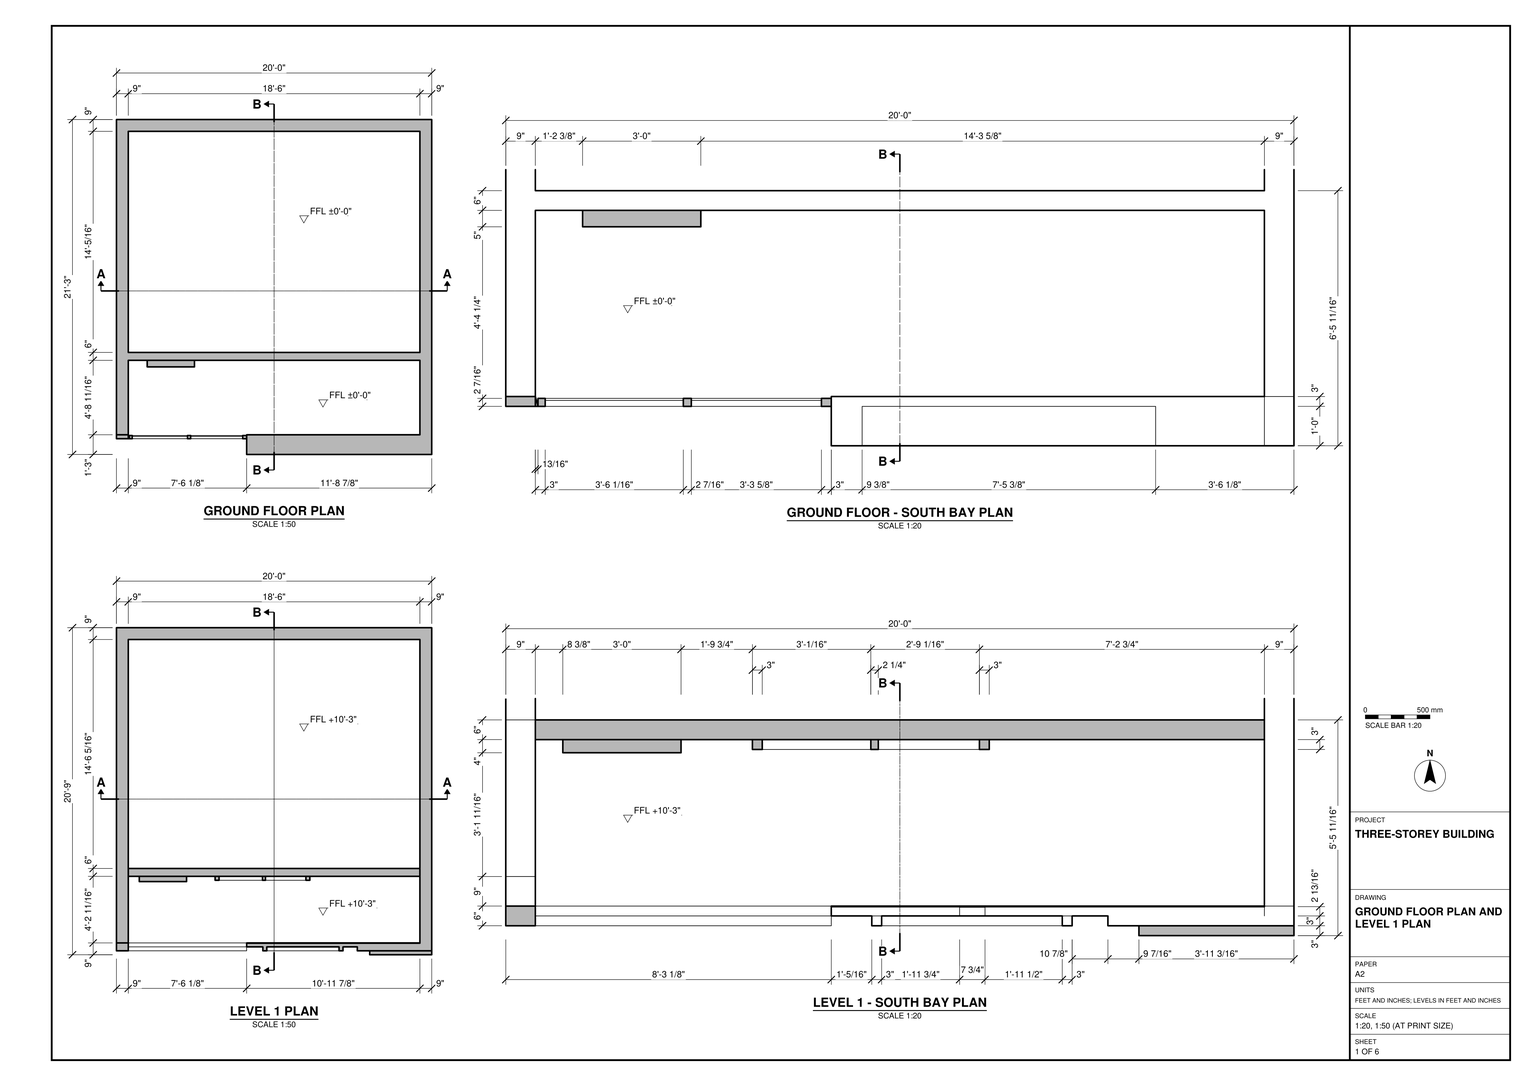
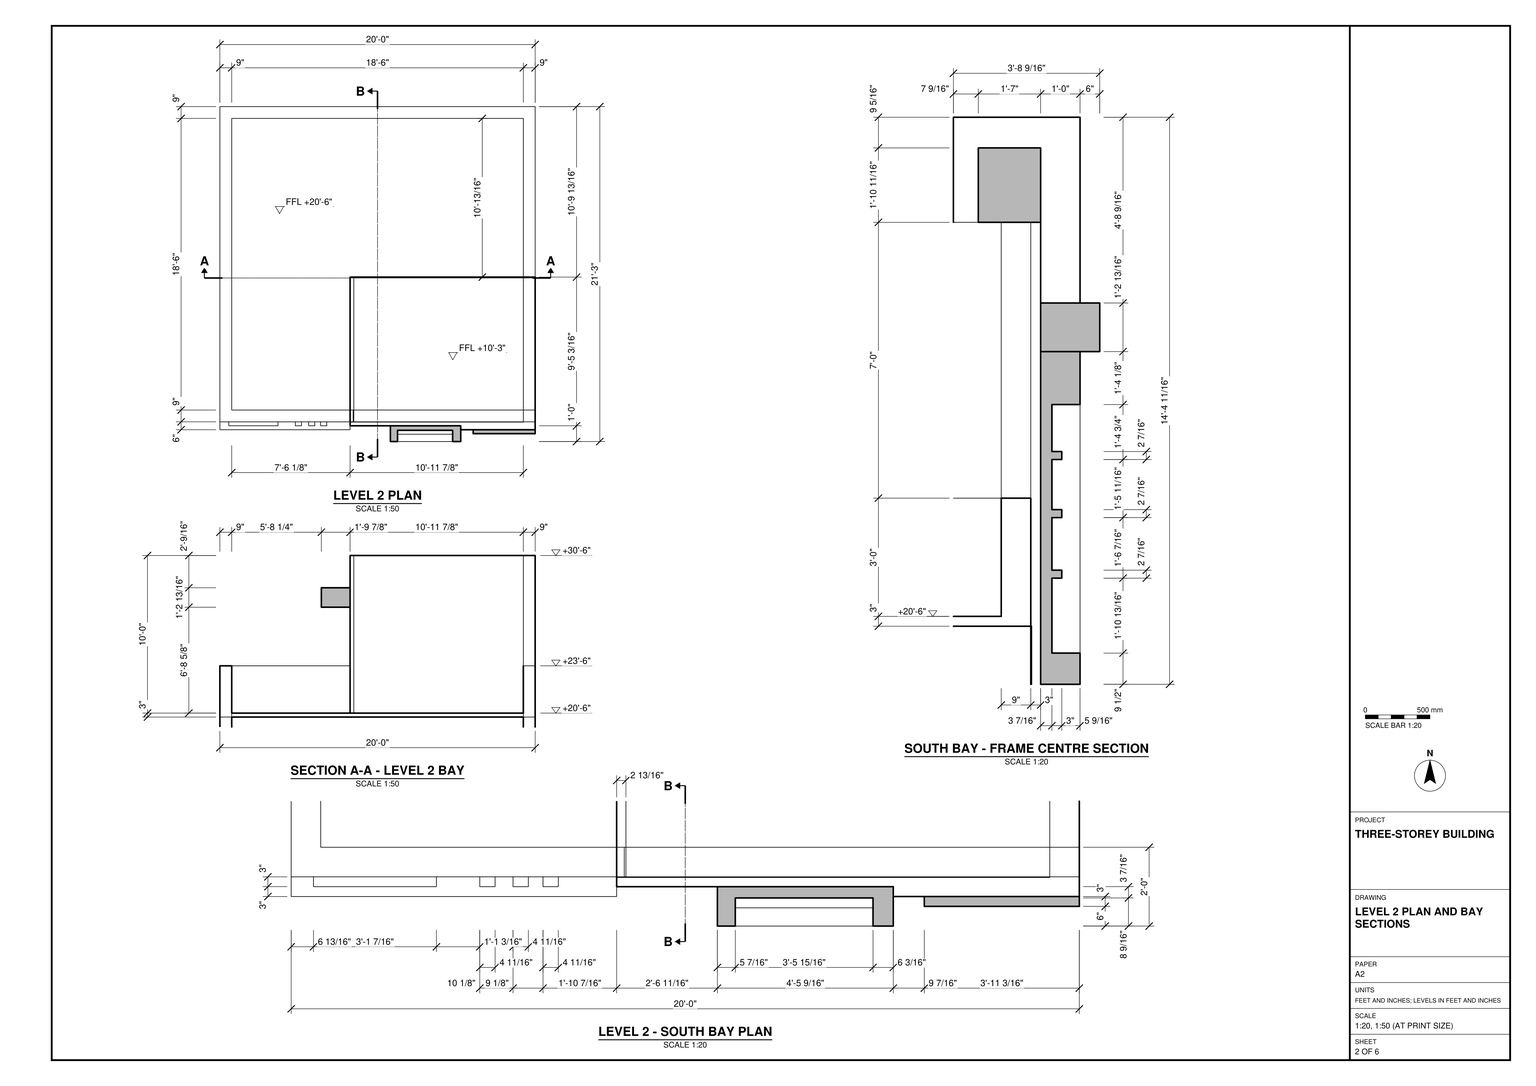
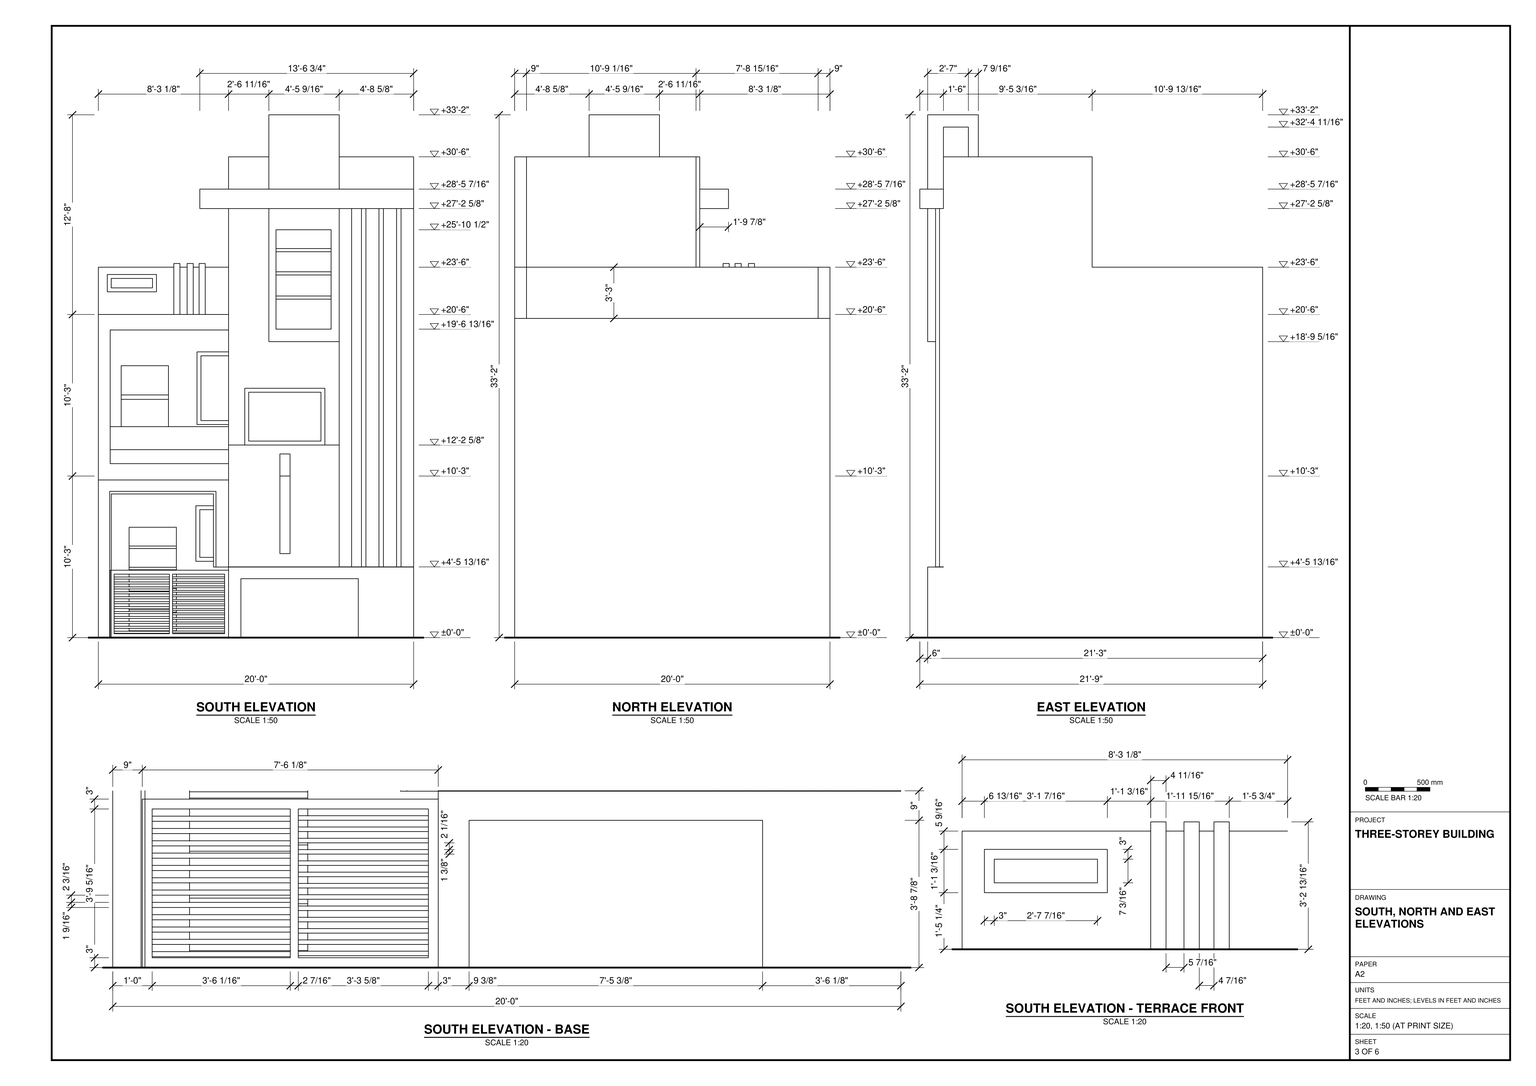
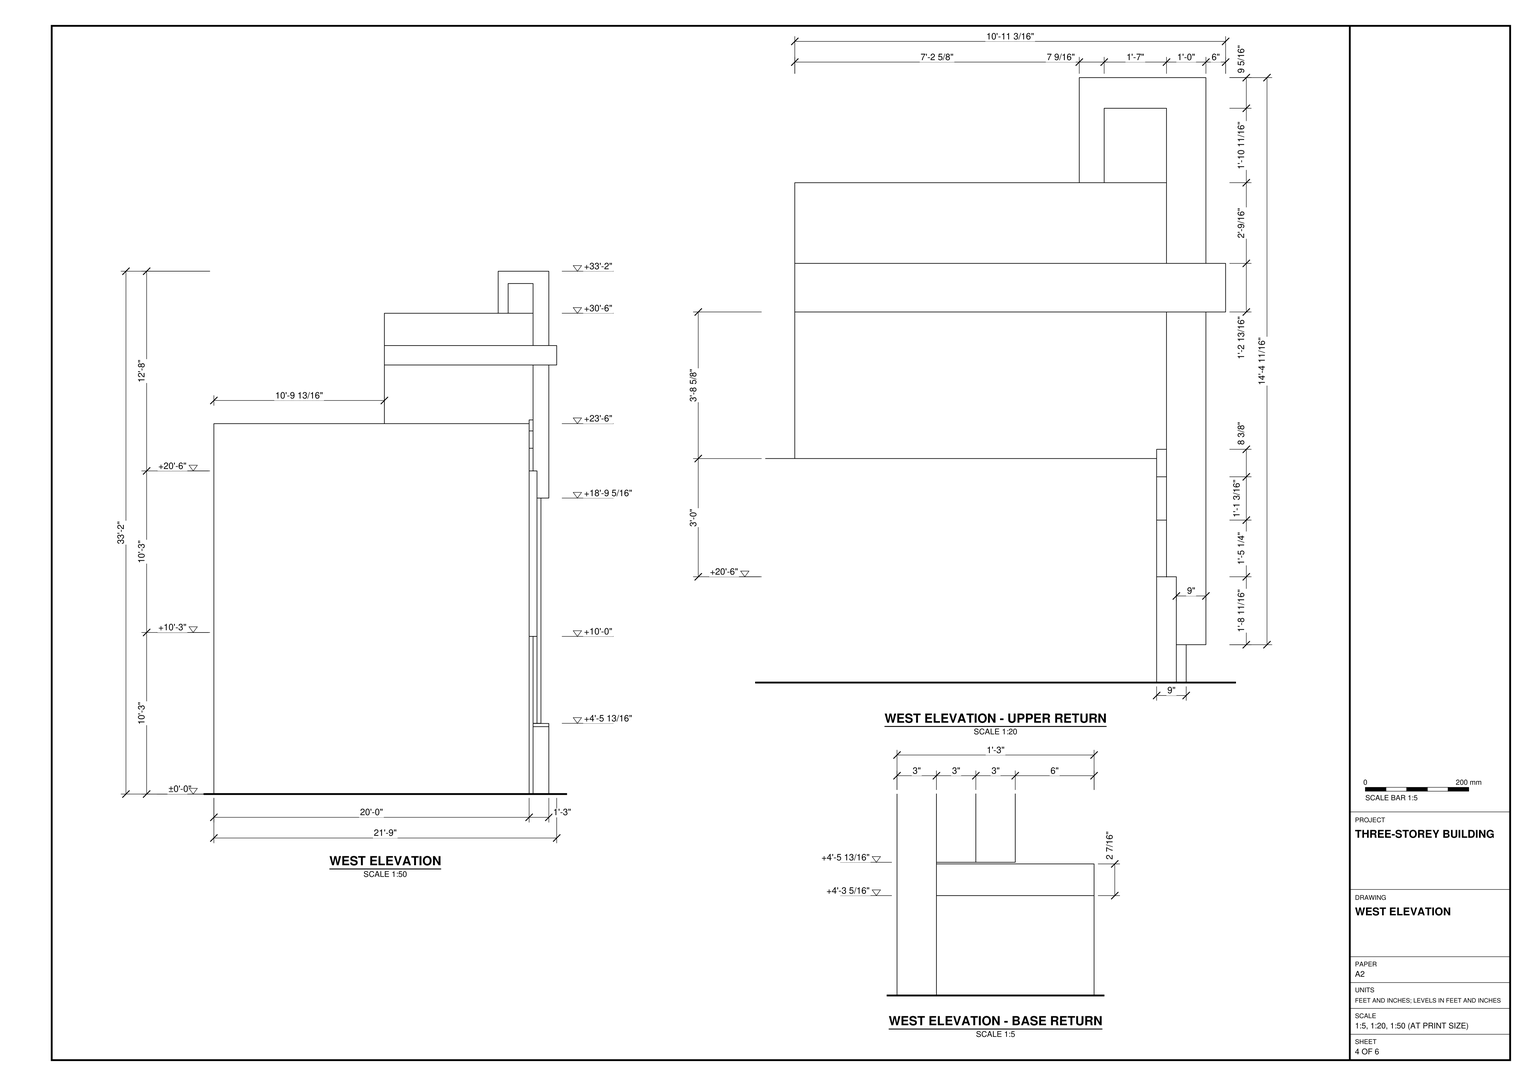
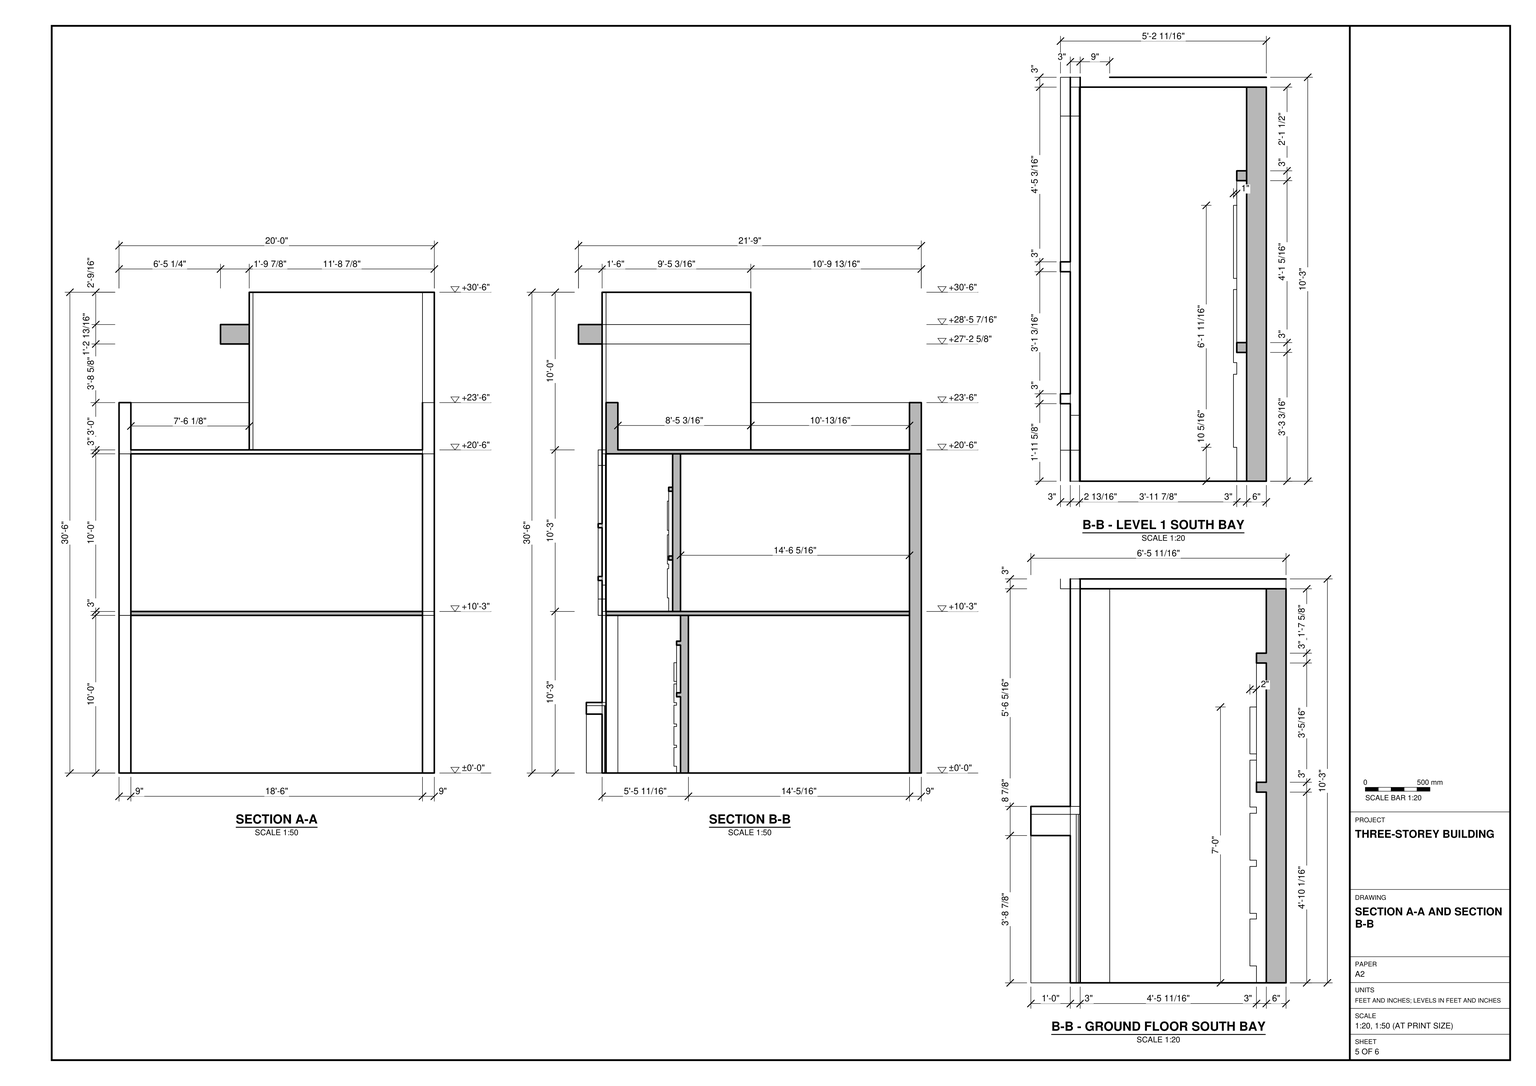
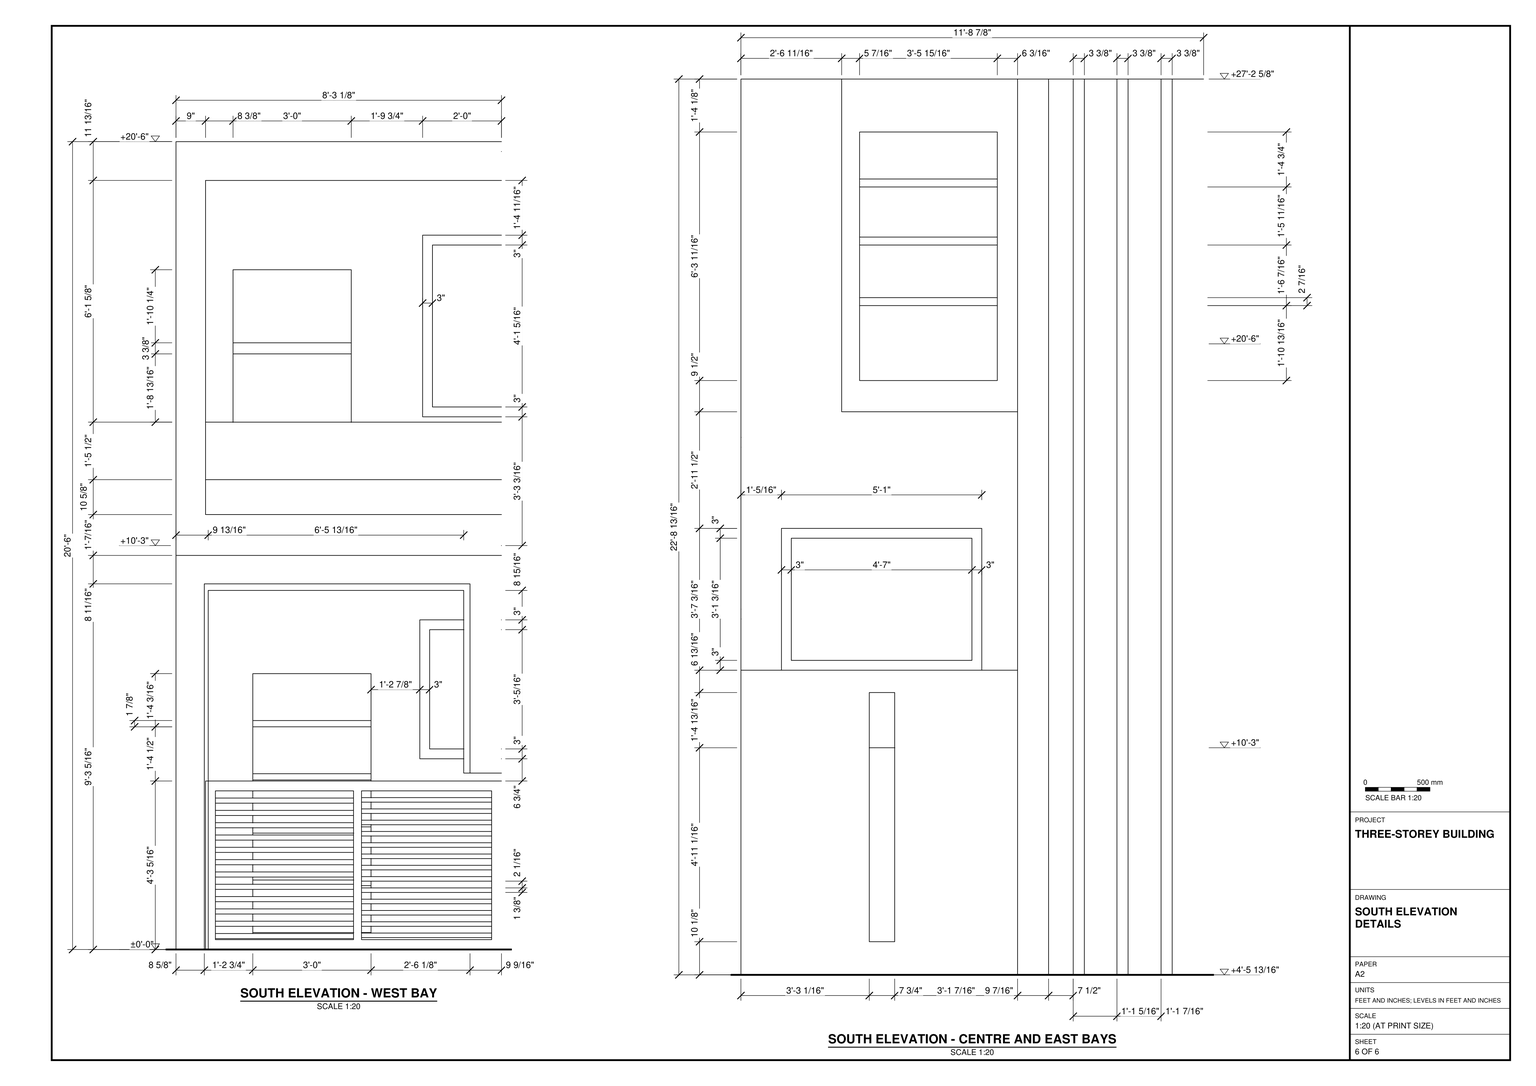
Build the three-storey building in SketchUp from task_files/diagram_01.pdf. Work in feet and inches. Set the overall width to 20'-0", the depth including the south façade projections to 21'-9", and the height to 33'-2". Set the ground floor at ±0'-0", Level 1 at +10'-3", and Level 2 at +20'-6".

Use the floor plans to lay out the main enclosure and the shallow bay along its south side. Model the 9" perimeter walls and the 6" transverse walls where dimensioned. Follow the sections for the floor slabs, flat roof, terrace parapet and taller volume at the southeast corner. Use the enlarged bay plans with the south elevation to place the openings, frames and projections at their correct depths. On the left, model the slatted gate and the recessed bays behind and above it. On the right, include the solid base, tall vertical fins, raised rectangular frame and projecting horizontal band. Carry the terrace-front details around only as far as the plans show.

Keep walls, slabs and roof elements in separate groups or components, and do the same for each furniture or joinery piece shown. Use components for repeated parts. Decor and loose items may be any suitable library components. Save one SketchUp model as output_files/three_storey_building_with_a_recessed_south_bay.skp.

# SketchUp Ruby script. Lengths in inches.
U = 1.inch
M = Sketchup.active_model
def pt(a) = Geom::Point3d.new(a.map { |v| v * U })
def face(e, loops, mat)
  f = e.add_face(loops[0].map { |a| pt(a) })
  loops[1..].each { |l| e.add_face(l.map { |a| pt(a) }).erase! }
  f.material = f.back_material = mat if mat
  f
end
# faces: each face lists its corners as indices into pts; further lists are holes
def faces(e, pts, list, mat = nil) = list.each { |f| face(e, (f[0].is_a?(Array) ? f : [f]).map { |l| l.map { |i| pts[i] } }, mat) }
# xy, xz, yz: faces in a plane at the given z, y or x. An outline is a flat list of corners, or four numbers for a rectangle; further outlines are holes
def ring(l) = l.size == 4 ? [[l[0], l[1]], [l[2], l[1]], [l[2], l[3]], [l[0], l[3]]] : l.each_slice(2).to_a
def flat(e, list, mat, &to3) = list.each { |f| face(e, (f[0].is_a?(Array) ? f : [f]).map { |l| ring(l).map { |u, v| to3.(u, v) } }, mat) }
def xy(e, z, list, mat = nil) = flat(e, list, mat) { |x, y| [x, y, z] }
def xz(e, y, list, mat = nil) = flat(e, list, mat) { |x, z| [x, y, z] }
def yz(e, x, list, mat = nil) = flat(e, list, mat) { |y, z| [x, y, z] }
def lines(e, pts, list) = list.each { |a, b| e.add_line(pt(pts[a]), pt(pts[b])) }
# prism: a flat outline (further loops are holes) pulled along v
def prism(e, loops, v, mat = nil)
  f = face(e, loops, mat); d = Geom::Vector3d.new(v.map { |x| x * U })
  f.pushpull(f.normal.samedirection?(d) ? d.length : -d.length)
end
def box(e, o, s, mat = nil) = prism(e, [[o, [o[0] + s[0], o[1], o[2]], [o[0] + s[0], o[1] + s[1], o[2]], [o[0], o[1] + s[1], o[2]]]], [0, 0, s[2]], mat)
def at(x, y, z, deg = 0) = Geom::Transformation.translation(pt([x, y, z])) * Geom::Transformation.rotation(ORIGIN, Z_AXIS, deg.degrees)
def axes(o, x, y, z) = Geom::Transformation.new([*x, 0, *y, 0, *z, 0, *pt(o).to_a, 1])
def part(name) = M.definitions.add(name)
# library, detail: a bought-in or finely detailed component or shape, given as its bounding box
def library(name, o, s) = part(name).tap { |d| box(d.entities, o, s) }
def detail(e, o, s) = box(e.add_group.entities, o, s)
def put(e, d, t, mat = nil) = e.add_instance(d, t).tap { |i| i.material = mat if mat }
def group(e, t, mat = nil) = e.add_group.tap { |g| g.transformation = t; g.material = mat if mat }.entities
root = M.entities
M.materials.add("[0004_HotPink]").color = [193, 79, 136]
M.materials.add("[0022_Maroon]").color = [128, 0, 0]
M.materials.add("[0079_Teal]").color = [0, 104, 104]
M.materials.add("[Color B07]").color = [153, 38, 0]
M.materials.add("[Color B08]").color = [63, 15, 0]
M.materials.add("[Color H08]").color = [0, 102, 102]
M.materials.add("[Color L03]").color = [206, 81, 144]
M.materials.add("[Color M05]").color = [114, 114, 114]
M.materials.add("[Color M09]").color = [0, 0, 0]
M.materials.add("[Formica Beige]").color = [211, 187, 149]
M.materials.add("[Formica Speckled Grey]").color = [94, 105, 111]
M.materials.add("[Translucent Glass Blue]").color = [67, 100, 160]
M.materials["[Translucent Glass Blue]"].alpha = 0.5
M.materials.add("[Translucent Glass Gray]").color = [198, 161, 76]
M.materials["[Translucent Glass Gray]"].alpha = 0.5
M.materials.add("[Wood Floor Parquet]").color = [122, 75, 32]
xy(root,0,[[99.11,6,99.11,21,231,21,231,6,197.89,6,197.89,18,108.51,18,108.51,6],[231,6,240,21],[0,18,9,21],[9,18,9,21,9.32,19.8125,9.32,18],[9.81,18,9.81,20.4375,99.11,20.4375,99.11,21,231,21,231,77.6875,59.39,77.6875,59.39,74.6875,23.39,74.6875,23.39,77.6875,9,77.6875,9,21,9.32,19.8125],
  [9.32,18,9.32,19.8125,9.81,18],[9.81,18,99.11,19.8125],[9.81,19.8125,99.11,20.4375],[[0,21,0,261,240,261,240,21,231,21,231,77.6875,9,77.6875,9,21],[9,83.6875,231,252]],[23.39,74.6875,59.39,77.6875],
  [9,83.6875,231,252]])
xy(root,3,[[12,19.8125,54.06,20.4375],[56.5,19.8125,96.11,20.4375]])
xy(root,3,[[12,18,54.06,19.8125],[56.5,18,96.11,19.8125]],"[Color M09]")
xy(root,5.15,[[23.39,72.6875,59.39,74.6875]])
xy(root,19.4375,[[23.39,72.6875,59.39,74.6875]],"[Color B08]")
xy(root,21.15,[[23.39,72.6875,59.39,74.6875]],"[Color B08]")
xy(root,34.86,[[12,19.8125,54.06,20.4375]])
xy(root,35.4375,[[23.39,72.6875,59.39,74.6875]],"[Color B08]")
xy(root,37.06,[[12,19.8125,54.06,20.4375]])
xy(root,37.34,[[23.39,72.6875,59.39,74.6875]],"[Color B08]")
xy(root,38.61,[[12,19.8125,54.06,20.4375]])
xy(root,40.81,[[12,19.8125,54.06,20.4375]])
xy(root,42.36,[[12,19.8125,54.06,20.4375]])
xy(root,44.56,[[12,19.8125,54.06,20.4375]])
xy(root,44.85,[[108.51,6,197.89,18]])
xy(root,46.11,[[12,19.8125,54.06,20.4375]])
xy(root,48.31,[[56.5,19.8125,96.11,20.4375]])
xy(root,48.31,[[12,18,54.06,20.4375],[56.5,18,96.11,19.8125]],"[Color M09]")
xy(root,51.31,[[9,18,9.81,18,9.81,20.4375,99.11,20.4375,99.11,21,9,21]])
xy(root,51.31,[[9.81,18,99.11,20.4375]],"[Color M09]")
xy(root,51.625,[[23.39,72.6875,59.39,74.6875]],"[Color B08]")
xy(root,53.53,[[23.39,72.6875,59.39,74.6875]],"[Color B08]")
xy(root,53.72,[[99.11,6,240,18],[87.61,18,99.11,21]])
xy(root,53.84,[[192.79,12,240,15],[183.35,15,240,18]])
xy(root,58.07,[[74.24,74.6875,126.74,77.6875]],"[Color B07]")
xy(root,61.07,[[77.24,74.6875,100.49,77.6875],[102.23,74.6875,123.74,77.6875]],"[Color B07]")
xy(root,63.9375,[[138.2,18,145.93,20.625]],"[Color L03]")
xy(root,67.8125,[[23.39,72.6875,59.39,74.6875]],"[Color B08]")
xy(root,69.72,[[23.39,72.6875,59.39,74.6875]],"[Color B08]")
xy(root,84,[[23.39,72.6875,59.39,77.6875]],"[Color B08]")
xy(root,97.39,[[77.24,74.6875,100.49,77.6875],[102.23,74.6875,123.74,77.6875]],"[Color B07]")
xy(root,100.39,[[74.24,74.6875,126.74,77.6875]],"[Color B07]")
xy(root,109.34,[[9.81,18,9,21,87.61,21,87.61,18]])
xy(root,120,[[0,15,9,18],[9,15,99.11,18],[0,18,99.11,21],[9,21,231,77.6875],[9,77.6875,231,83.6875],
  [9,83.6875,231,252]])
xy(root,123,[[99.11,20.8125,231,21],[9,21,231,21,231,71.6875,53.37,71.6875,53.37,68.6875,17.37,68.6875,17.37,71.6875,9,71.6875],[17.37,68.6875,53.37,71.6875],[9,71.6875,231,77.6875],[9,77.6875,231,252]])
xy(root,132.44,[[9,15,99.11,18],[9,18,99.11,21]])
xy(root,133.3125,[[17.37,67.6875,53.37,68.6875]])
xy(root,139.82,[[138.2,18,145.93,20.625]],"[Color L03]")
xy(root,143.07,[[9,18,99.11,21]])
xy(root,146.61,[[111.45,15,172.45,18]])
xy(root,149.61,[[114.45,15,169.45,18]])
xy(root,155.5625,[[17.37,67.6875,53.37,68.6875]],"[Color B08]")
xy(root,159.125,[[17.37,67.6875,53.37,68.6875]])
xy(root,162.21,[[75.1,68.6875,147.22,71.6875]])
xy(root,165.21,[[78.1,68.6875,111.16,71.6875],[113.44,68.6875,144.22,71.6875]],"[Color B07]")
xy(root,181.375,[[17.37,67.6875,53.37,68.6875]],"[Color B08]")
xy(root,184.75,[[17.37,67.6875,53.37,68.6875]],"[Color B08]")
xy(root,186.8,[[114.45,15,169.45,18]])
xy(root,189.8,[[111.45,15,172.45,18]])
xy(root,207,[[17.37,67.6875,53.37,71.6875]],"[Color B08]")
xy(root,214.52,[[78.1,68.6875,111.16,71.6875],[113.44,68.6875,144.22,71.6875]],"[Color B07]")
xy(root,217.52,[[75.1,68.6875,147.22,71.6875]],"[Color B07]")
xy(root,225.3125,[[129.79,6,183.35,18]],"[Color L03]")
xy(root,234.1875,[[9,15,99.11,21]])
xy(root,234.82,[[135.24,6,177.18,14.5625]],"[Color L03]")
xy(root,243,[[99.11,20.8125,231,21],[9,21,231,71.6875],[9,71.6875,231,77.6875],[9,77.6875,231,252],[9,252,231,252.125],
  [9,252.125,231,261]])
xy(root,246,[[0,15,99.11,15,99.11,21,81.35,21,81.35,18,76.69,18,76.69,21,72.22,21,72.22,18,67.56,18,67.56,21,62.1,21,62.1,18,57.44,18,57.44,21,0,21],[57.44,18,62.1,21],[67.56,18,72.22,21],[76.69,18,81.35,21],[9,30,99.11,30,99.11,131.1875,231,131.1875,231,252,9,252],
  [99.11,30,101.9375,131.1875],[101.9375,30,231,131.1875]])
xy(root,257.65,[[135.24,11.5625,177.18,14.5625]],"[0022_Maroon]")
xy(root,260.07,[[135.24,11.5625,177.18,14.5625]],"[0022_Maroon]")
xy(root,263.25,[[6.79,18,44.23,21]])
xy(root,266.25,[[9.79,18,41.23,30]])
xy(root,273.4375,[[9.79,18,41.23,30]])
xy(root,276.08,[[135.24,11.5625,177.18,14.5625]],"[0022_Maroon]")
xy(root,276.4375,[[6.79,18,44.23,21]])
xy(root,278.51,[[135.24,11.5625,177.18,14.5625]],"[0022_Maroon]")
xy(root,282,[[0,21,99.11,21,99.11,30,9,30,9,252,231,252,231,131.1875,240,131.1875,240,261,0,261],[99.11,21,101.4375,30],[101.4375,21,101.9375,30],[101.9375,21,231,30]])
xy(root,284.8125,[[57.44,18,62.1,21],[67.56,18,72.22,21],[76.69,18,81.35,21]],"[Formica Speckled Grey]")
xy(root,293.77,[[135.24,11.5625,177.18,14.5625]],"[0022_Maroon]")
xy(root,296.2,[[135.24,11.5625,177.18,14.5625]],"[0022_Maroon]")
xy(root,310.51,[[135.24,6,177.18,14.5625]],"[Color L03]")
xy(root,326.63,[[77.24,0,77.24,131.1875,99.11,131.1875,99.11,18,129.79,18,129.79,6,183.35,6,183.35,15,192.79,15,192.79,12,240,12,240,0],[129.79,6,183.35,18],[192.79,12,240,15],[183.35,15,240,18]])
xy(root,341.43,[[77.24,0,240,0,240,18,183.35,18,183.35,6,129.79,6,129.79,18,99.11,18,99.11,131.1875,77.24,131.1875],[129.79,6,183.35,18]])
xy(root,366,[[[99.11,18,240,131.1875],[129.79,36.98,183.35,44.5625]]],"[0079_Teal]")
xy(root,388.66,[[129.79,18,183.35,36.98]],"[0004_HotPink]")
xy(root,398,[[129.79,6,183.35,44.5625]],"[0004_HotPink]")
xz(root,0,[[77.24,326.63,240,341.43]])
xz(root,6,[[99.11,0,108.51,0,108.51,44.85,197.89,44.85,197.89,0,240,0,240,53.72,99.11,53.72]])
xz(root,6,[[[129.79,225.3125,183.35,326.63],[135.24,234.82,177.18,310.51]],[129.79,341.43,183.35,398]],"[Color L03]")
xz(root,11.5625,[[135.24,257.65,177.18,260.07],[135.24,276.08,177.18,278.51],[135.24,293.77,177.18,296.2]],"[0022_Maroon]")
xz(root,12,[[200.3,53.84,203.68,326.63],[213.61,53.84,216.99,326.63],[227.05,53.84,230.43,326.63]])
xz(root,12,[[192.79,53.84,200.3,326.63],[203.68,53.84,213.61,326.63],[216.99,53.84,227.05,326.63],[230.43,53.84,240,326.63]],"[Color M05]")
xz(root,14.5625,[[135.24,234.82,177.18,257.65],[135.24,260.07,177.18,276.08],[135.24,278.51,177.18,293.77],[135.24,296.2,177.18,310.51]],"[Translucent Glass Blue]")
xz(root,15,[[192.79,53.84,240,326.63],[0,120,99.11,120,99.11,132.44,9,132.44,9,234.1875,99.11,234.1875,99.11,246,0,246],[[111.45,146.61,172.45,189.8],[114.45,149.61,169.45,186.8]]])
xz(root,15,[[183.35,53.84,192.79,326.63]],"[Color M05]")
xz(root,18,[[8.62,0,9,0,9,51.31,9.81,51.31,9.81,109.34,87.61,109.34,87.61,53.72,89.53,53.72,89.53,111.34,8.62,111.34],[9,0,9.81,51.31],[99.11,53.72,108.51,53.84],[108.51,53.72,240,53.84],[114.45,149.61,169.45,186.8],
  [129.79,225.3125,183.35,326.63],[[6.79,263.25,44.23,276.4375],[9.79,266.25,41.23,273.4375]],[99.11,326.63,129.79,341.43],[129.79,326.63,183.35,341.43],[183.35,326.63,240,341.43],
  [129.79,341.43,183.35,366]])
xz(root,18,[[129.79,366,183.35,388.66]],"[0004_HotPink]")
xz(root,18,[[99.11,146.61,111.45,146.61,111.45,189.8,172.45,189.8,172.45,146.61,183.35,146.61,183.35,225.3125,129.79,225.3125,129.79,326.63,99.11,326.63],[99.11,341.43,129.79,366],[183.35,341.43,240,366]],"[0079_Teal]")
xz(root,18,[[0,0,8.62,0,8.62,111.34,89.53,111.34,89.53,53.72,99.11,53.72,99.11,120,0,120]],"[Color H08]")
xz(root,18,[[[99.11,53.84,183.35,146.61],[138.2,63.9375,145.93,139.82]]],"[Color L03]")
xz(root,18,[[[9.81,0,99.11,51.31],[12,3,54.06,48.31],[56.5,3,96.11,48.31]]],"[Color M09]")
xz(root,18,[[57.44,246,62.1,284.8125],[67.56,246,72.22,284.8125],[76.69,246,81.35,284.8125]],"[Formica Speckled Grey]")
xz(root,18,[[9,143.07,99.11,160.59]],"[Translucent Glass Blue]")
xz(root,18,[[108.51,0,197.89,44.85],[9,132.44,99.11,143.07]],"[Wood Floor Parquet]")
xz(root,19.8125,[[12,1.11,54.06,3],[56.5,1.5625,96.11,3],[12,3,54.06,3.31],[56.5,3,96.11,3.62],[12,3.31,54.06,4.86],
  [56.5,3.62,96.11,5],[12,7.06,54.06,8.61],[56.5,7.06,96.11,8.4375],[56.5,10.49,96.11,11.875],[12,10.81,54.06,12.36],
  [56.5,13.93,96.11,15.3125],[12,14.56,54.06,16.11],[56.5,17.37,96.11,18.75],[12,18.31,54.06,19.86],[56.5,20.81,96.11,22.1875],
  [12,22.06,54.06,23.61],[56.5,24.24,96.11,25.625],[12,25.81,54.06,27.36],[56.5,27.68,96.11,29.0625],[12,29.56,54.06,31.11],
  [56.5,31.12,96.11,32.5],[12,33.31,54.06,34.86],[56.5,34.56,96.11,35.9375],[12,37.06,54.06,38.61],[56.5,37.99,96.11,39.375],
  [12,40.81,54.06,42.36],[56.5,41.43,96.11,42.8125],[12,44.56,54.06,46.11],[56.5,44.87,96.11,46.25]])
xz(root,20.4375,[[[9.81,0,99.11,51.31],[12,3,54.06,48.31],[56.5,3,96.11,48.31]]])
xz(root,20.625,[[138.2,63.9375,145.93,139.82]])
xz(root,20.8125,[[99.11,123,231,243]])
xz(root,21,[[0,0,9,120],[99.11,0,231,120],[87.61,53.72,99.11,109.34],[0,120,9,242.93],[9,120,99.11,123],
  [99.11,120,231,123],[9,123,99.11,132.44],[99.11,123,231,243],[9,132.44,99.11,143.07],[9,234.1875,99.11,242.93],
  [0,242.93,0,246,99.11,246,99.11,243,9,243,9,242.93],[9,242.93,99.11,243],[99.11,243,231,282],[57.44,246,62.1,282],[67.56,246,72.22,282],
  [76.69,246,81.35,282],[57.44,282,62.1,284.8125],[67.56,282,72.22,284.8125],[76.69,282,81.35,284.8125]])
xz(root,21,[[[0,246,57.44,282],[6.79,263.25,44.23,276.4375]],[62.1,246,67.56,282],[72.22,246,76.69,282],[81.35,246,99.11,282]],"[Formica Beige]")
xz(root,30,[[[9,246,99.11,282],[9.79,266.25,41.23,273.4375]],[99.11,246,101.9375,282],[101.9375,246,231,282]])
xz(root,36.98,[[129.79,366,183.35,388.66]],"[0004_HotPink]")
xz(root,44.5625,[[129.79,366,183.35,398]])
xz(root,67.6875,[[17.37,133.3125,53.37,155.5625],[17.37,159.125,53.37,181.375],[17.37,184.75,53.37,207]],"[Color B08]")
xz(root,68.6875,[[[75.1,162.21,147.22,217.52],[78.1,165.21,111.16,214.52],[113.44,165.21,144.22,214.52]]],"[Color B07]")
xz(root,68.6875,[[17.37,123,53.37,133.3125],[17.37,155.5625,53.37,159.125],[17.37,181.375,53.37,184.75]],"[Color B08]")
xz(root,71.6875,[[[9,123,17.37,123,17.37,207,53.37,207,53.37,123,231,123,231,243,9,243],[75.1,162.21,147.22,217.52]],[17.37,123,53.37,207],[[75.1,162.21,147.22,217.52],[78.1,165.21,111.16,214.52],[113.44,165.21,144.22,214.52]]])
xz(root,71.6875,[[78.1,165.21,111.16,214.52],[113.44,165.21,144.22,214.52]],"[Translucent Glass Gray]")
xz(root,72.6875,[[23.39,5.15,59.39,19.4375],[23.39,21.15,59.39,35.4375],[23.39,37.34,59.39,51.625],[23.39,53.53,59.39,67.8125],[23.39,69.72,59.39,84]],"[Color B08]")
xz(root,74.6875,[[[74.24,58.07,126.74,100.39],[77.24,61.07,100.49,97.39],[102.23,61.07,123.74,97.39]]],"[Color B07]")
xz(root,74.6875,[[23.39,0,59.39,5.15],[23.39,19.4375,59.39,21.15],[23.39,35.4375,59.39,37.34],[23.39,51.625,59.39,53.53],[23.39,67.8125,59.39,69.72]],"[Color B08]")
xz(root,77.6875,[[[9,0,23.39,0,23.39,84,59.39,84,59.39,0,231,0,231,120,9,120],[74.24,58.07,126.74,100.39]],[23.39,0,59.39,84],[9,123,231,243]])
xz(root,77.6875,[[77.24,61.07,100.49,97.39],[102.23,61.07,123.74,97.39]],"[Translucent Glass Gray]")
xz(root,83.6875,[[9,0,231,120]])
xz(root,131.1875,[[99.11,246,101.9375,366],[77.24,326.63,99.11,341.43]])
xz(root,131.1875,[[101.9375,246,231,366],[231,282,240,366]],"[0079_Teal]")
xz(root,252,[[9,0,231,120],[9,120,231,123],[9,123,231,243],[9,246,231,282]])
xz(root,261,[[0,0,240,243],[0,243,9,282],[9,243,231,282],[231,243,240,282]])
yz(root,0,[[18,0,21,120],[21,0,261,282],[15,120,21,246]])
yz(root,6.79,[[18,263.25,21,276.4375]])
yz(root,9,[[18,0,21,51.31],[21,0,30,120],[30,0,77.6875,120],[83.6875,0,252,120],[21,120,83.6875,123],
  [83.6875,120,252,123],[21,123,71.6875,243],[71.6875,123,77.6875,243],[77.6875,123,252,243],[15,132.44,18,132.44,18,143.07,21,143.07,21,234.1875,15,234.1875],
  [18,132.44,21,143.07],[252,243,252.125,246],[252.125,243,261,246],[30,246,252,282]])
yz(root,9.79,[[18,266.25,30,273.4375]])
yz(root,9.81,[[18,0,19.8125,51.31],[19.8125,0,20.4375,51.31]])
yz(root,12,[[19.8125,3,20.4375,34.86],[19.8125,37.06,20.4375,38.61],[19.8125,40.81,20.4375,42.36],[19.8125,44.56,20.4375,46.11]])
yz(root,12,[[18,3,19.8125,3,19.8125,34.86,20.4375,34.86,20.4375,37.06,19.8125,37.06,19.8125,38.61,20.4375,38.61,20.4375,40.81,19.8125,40.81,19.8125,42.36,20.4375,42.36,20.4375,44.56,19.8125,44.56,19.8125,46.11,20.4375,46.11,20.4375,48.31,18,48.31]],"[Color M09]")
yz(root,17.37,[[68.6875,123,68.6875,133.3125,67.6875,133.3125,67.6875,155.5625,68.6875,155.5625,68.6875,159.125,67.6875,159.125,67.6875,181.375,68.6875,181.375,68.6875,184.75,67.6875,184.75,67.6875,207,71.6875,207,71.6875,123]],"[Color B08]")
yz(root,23.39,[[74.6875,0,74.6875,5.15,72.6875,5.15,72.6875,19.4375,74.6875,19.4375,74.6875,21.15,72.6875,21.15,72.6875,35.4375,74.6875,35.4375,74.6875,37.34,72.6875,37.34,72.6875,51.625,74.6875,51.625,74.6875,53.53,72.6875,53.53,72.6875,67.8125,74.6875,67.8125,74.6875,69.72,72.6875,69.72,72.6875,84,77.6875,84,77.6875,0]],"[Color B08]")
yz(root,41.23,[[18,266.25,30,273.4375]])
yz(root,44.23,[[18,263.25,21,276.4375]])
yz(root,53.37,[[68.6875,123,71.6875,123,71.6875,207,67.6875,207,67.6875,184.75,68.6875,184.75,68.6875,181.375,67.6875,181.375,67.6875,159.125,68.6875,159.125,68.6875,155.5625,67.6875,155.5625,67.6875,133.3125,68.6875,133.3125]],"[Color B08]")
yz(root,54.06,[[19.8125,3,20.4375,34.86],[19.8125,37.06,20.4375,38.61],[19.8125,40.81,20.4375,42.36],[19.8125,44.56,20.4375,46.11]])
yz(root,54.06,[[18,3,18,48.31,20.4375,48.31,20.4375,46.11,19.8125,46.11,19.8125,44.56,20.4375,44.56,20.4375,42.36,19.8125,42.36,19.8125,40.81,20.4375,40.81,20.4375,38.61,19.8125,38.61,19.8125,37.06,20.4375,37.06,20.4375,34.86,19.8125,34.86,19.8125,3]],"[Color M09]")
yz(root,56.5,[[19.8125,3,20.4375,48.31]])
yz(root,56.5,[[18,3,19.8125,48.31]],"[Color M09]")
yz(root,57.44,[[18,246,21,284.8125]],"[Formica Speckled Grey]")
yz(root,59.39,[[74.6875,0,77.6875,0,77.6875,84,72.6875,84,72.6875,69.72,74.6875,69.72,74.6875,67.8125,72.6875,67.8125,72.6875,53.53,74.6875,53.53,74.6875,51.625,72.6875,51.625,72.6875,37.34,74.6875,37.34,74.6875,35.4375,72.6875,35.4375,72.6875,21.15,74.6875,21.15,74.6875,19.4375,72.6875,19.4375,72.6875,5.15,74.6875,5.15]],"[Color B08]")
yz(root,62.1,[[18,246,21,284.8125]],"[Formica Speckled Grey]")
yz(root,67.56,[[18,246,21,284.8125]],"[Formica Speckled Grey]")
yz(root,72.22,[[18,246,21,284.8125]],"[Formica Speckled Grey]")
yz(root,74.24,[[74.6875,58.07,77.6875,100.39]],"[Color B07]")
yz(root,75.1,[[68.6875,162.21,71.6875,217.52]],"[Color B07]")
yz(root,76.69,[[18,246,21,284.8125]],"[Formica Speckled Grey]")
yz(root,77.24,[[0,326.63,131.1875,341.43]])
yz(root,77.24,[[74.6875,61.07,77.6875,97.39]],"[Color B07]")
yz(root,78.1,[[68.6875,165.21,71.6875,214.52]],"[Color B07]")
yz(root,81.35,[[18,246,21,284.8125]],"[Formica Speckled Grey]")
yz(root,87.61,[[18,53.72,21,109.34]])
yz(root,96.11,[[19.8125,3,20.4375,48.31]])
yz(root,96.11,[[18,3,19.8125,48.31]],"[Color M09]")
yz(root,99.11,[[6,0,18,51.31],[18,0,19.8125,51.31],[19.8125,0,20.4375,51.31],[20.4375,0,21,51.31],[6,51.31,18,53.72],
  [18,51.31,21,53.72],[18,53.72,21,120],[15,120,18,132.44],[18,120,21,123],[18,123,20.8125,132.44],
  [20.8125,123,21,132.44],[18,132.44,20.8125,143.07],[20.8125,132.44,21,143.07],[18,143.07,20.8125,234.1875],[20.8125,143.07,21,234.1875],
  [15,234.1875,18,246],[18,234.1875,20.8125,243],[20.8125,234.1875,21,243],[18,243,21,246],[18,326.63,131.1875,341.43]])
yz(root,99.11,[[18,246,18,326.63,131.1875,326.63,131.1875,246,30,246,30,282,21,282,21,246],[18,341.43,131.1875,366]],"[0079_Teal]")
yz(root,100.49,[[74.6875,61.07,77.6875,97.39]],"[Color B07]")
yz(root,102.23,[[74.6875,61.07,77.6875,97.39]])
yz(root,108.51,[[6,0,18,44.85]])
yz(root,111.16,[[68.6875,165.21,71.6875,214.52]],"[Color B07]")
yz(root,111.45,[[15,146.61,18,189.8]])
yz(root,113.44,[[68.6875,165.21,71.6875,214.52]],"[Color B07]")
yz(root,114.45,[[15,149.61,18,186.8]])
yz(root,123.74,[[74.6875,61.07,77.6875,97.39]],"[Color B07]")
yz(root,126.74,[[74.6875,58.07,77.6875,100.39]])
yz(root,129.79,[[6,341.43,6,398,44.5625,398,44.5625,366,36.98,366,36.98,388.66,18,388.66,18,341.43]],"[0004_HotPink]")
yz(root,129.79,[[6,225.3125,18,326.63]],"[Color L03]")
yz(root,135.24,[[6,234.82,14.5625,234.82,14.5625,257.65,11.5625,257.65,11.5625,260.07,14.5625,260.07,14.5625,276.08,11.5625,276.08,11.5625,278.51,14.5625,278.51,14.5625,293.77,11.5625,293.77,11.5625,296.2,14.5625,296.2,14.5625,310.51,6,310.51]],"[Color L03]")
yz(root,138.2,[[18,63.9375,20.625,139.82]],"[Color L03]")
yz(root,144.22,[[68.6875,165.21,71.6875,214.52]],"[Color B07]")
yz(root,145.93,[[18,63.9375,20.625,139.82]],"[Color L03]")
yz(root,147.22,[[68.6875,162.21,71.6875,217.52]])
yz(root,169.45,[[15,149.61,18,186.8]])
yz(root,172.45,[[15,146.61,18,189.8]])
yz(root,177.18,[[6,234.82,6,310.51,14.5625,310.51,14.5625,296.2,11.5625,296.2,11.5625,293.77,14.5625,293.77,14.5625,278.51,11.5625,278.51,11.5625,276.08,14.5625,276.08,14.5625,260.07,11.5625,260.07,11.5625,257.65,14.5625,257.65,14.5625,234.82]],"[Color L03]")
yz(root,183.35,[[15,53.84,18,225.3125],[15,225.3125,18,326.63]])
yz(root,183.35,[[6,341.43,18,341.43,18,388.66,36.98,388.66,36.98,366,44.5625,366,44.5625,398,6,398]],"[0004_HotPink]")
yz(root,183.35,[[6,225.3125,15,326.63]],"[Color L03]")
yz(root,192.79,[[12,53.84,15,326.63]],"[Color M05]")
yz(root,197.89,[[6,0,18,44.85]])
yz(root,231,[[21,0,77.6875,120],[83.6875,0,252,120],[83.6875,120,252,123],[20.8125,123,21,243],[21,123,71.6875,243],
  [71.6875,123,77.6875,243],[77.6875,123,252,243],[30,246,131.1875,282],[131.1875,246,252,282]])
yz(root,240,[[6,0,261,0,261,282,131.1875,282,131.1875,366,18,366,18,326.63,15,326.63,15,53.84,18,53.84,18,53.72,6,53.72],[0,326.63,18,341.43]])
yz(root,240,[[12,53.84,15,326.63]],"[Color M05]")
p = [[9,21,109.34],[9.81,18,109.34],[9.81,18,51.31],[9.81,18,0],[9.32,19.8125,0],[9,21,0],
  [9,21,51.31],[9,252,120],[0,252,120],[9,77.6875,120],[0,77.6875,120],[9,30,120],
  [0,30,120],[231,252,120],[231,261,120],[231,252,123],[231,261,123],[9,261,120],
  [9,252,123],[9,261,123],[240,252,120],[240,252,123],[231,21,123],[240,21,123],
  [231,20.8125,123],[231,18,123],[56.5,19.8125,0.18],[96.11,19.8125,0.18],[231,21,282],[231,21,366],
  [231,30,282],[231,30,366],[240,21,282],[240,30,282],[101.4375,21,282],[101.4375,21,366],
  [101.9375,21,282],[101.9375,21,366]]
faces(root,p,[[0,1,2,3,4,5,6]])
lines(root,p,[[7,8],[9,10],[11,12],[13,14],[15,16],[7,17],[18,19],[13,20],[15,21],[22,23],[24,25],[26,27],
  [28,29],[30,31],[28,32],[30,33],[34,35],[36,37]])
